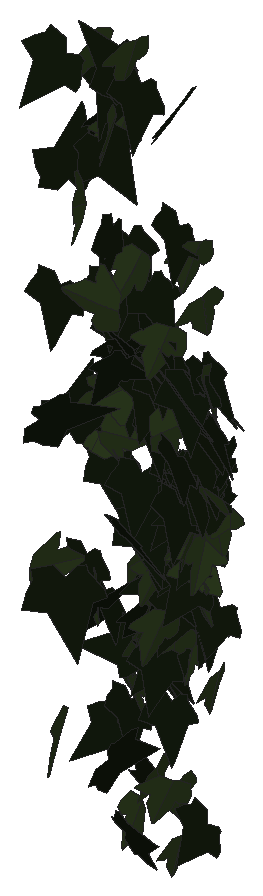
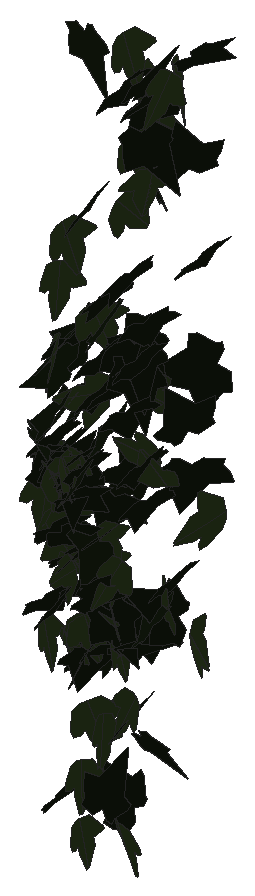
# SketchUp Ruby script. Lengths in inches.
U = 1.inch
M = Sketchup.active_model
def pt(a) = Geom::Point3d.new(a.map { |v| v * U })
def face(e, loops, mat)
  f = e.add_face(loops[0].map { |a| pt(a) })
  loops[1..].each { |l| e.add_face(l.map { |a| pt(a) }).erase! }
  f.material = f.back_material = mat if mat
  f
end
# faces: each face lists its corners as indices into pts; further lists are holes
def faces(e, pts, list, mat = nil) = list.each { |f| face(e, (f[0].is_a?(Array) ? f : [f]).map { |l| l.map { |i| pts[i] } }, mat) }
# xy, xz, yz: faces in a plane at the given z, y or x. An outline is a flat list of corners, or four numbers for a rectangle; further outlines are holes
def ring(l) = l.size == 4 ? [[l[0], l[1]], [l[2], l[1]], [l[2], l[3]], [l[0], l[3]]] : l.each_slice(2).to_a
def flat(e, list, mat, &to3) = list.each { |f| face(e, (f[0].is_a?(Array) ? f : [f]).map { |l| ring(l).map { |u, v| to3.(u, v) } }, mat) }
def xy(e, z, list, mat = nil) = flat(e, list, mat) { |x, y| [x, y, z] }
def xz(e, y, list, mat = nil) = flat(e, list, mat) { |x, z| [x, y, z] }
def yz(e, x, list, mat = nil) = flat(e, list, mat) { |y, z| [x, y, z] }
def lines(e, pts, list) = list.each { |a, b| e.add_line(pt(pts[a]), pt(pts[b])) }
# prism: a flat outline (further loops are holes) pulled along v
def prism(e, loops, v, mat = nil)
  f = face(e, loops, mat); d = Geom::Vector3d.new(v.map { |x| x * U })
  f.pushpull(f.normal.samedirection?(d) ? d.length : -d.length)
end
def box(e, o, s, mat = nil) = prism(e, [[o, [o[0] + s[0], o[1], o[2]], [o[0] + s[0], o[1] + s[1], o[2]], [o[0], o[1] + s[1], o[2]]]], [0, 0, s[2]], mat)
def at(x, y, z, deg = 0) = Geom::Transformation.translation(pt([x, y, z])) * Geom::Transformation.rotation(ORIGIN, Z_AXIS, deg.degrees)
def axes(o, x, y, z) = Geom::Transformation.new([*x, 0, *y, 0, *z, 0, *pt(o).to_a, 1])
def part(name) = M.definitions.add(name)
# library, detail: a bought-in or finely detailed component or shape, given as its bounding box
def library(name, o, s) = part(name).tap { |d| box(d.entities, o, s) }
def detail(e, o, s) = box(e.add_group.entities, o, s)
def put(e, d, t, mat = nil) = e.add_instance(d, t).tap { |i| i.material = mat if mat }
def group(e, t, mat = nil) = e.add_group.tap { |g| g.transformation = t; g.material = mat if mat }.entities
root = M.entities
M.materials.add("efeu1").color = [18, 25, 13]
M.materials.add("efeu2").color = [43, 57, 29]
c1 = part("ivyleaf_9")
p = [[1.54,2.16,1.25],[1.36,2.04,1.19],[-0.21,0.99,0.68],[-0.71,1.11,0.82],[-0.85,0.86,0.67],[-0.8,0.17,0.21],
  [-0.9,-0.01,0.1],[-0.67,-0.16,-0.02],[-0.08,-0.08,-0.05],[-0.03,-0.6,-0.4],[0.65,-0.88,-0.66],[0.83,-0.6,-0.49],
  [1.29,-0.42,-0.43],[1.8125,-0.07,-0.26],[1.21,0.44,0.15]]
faces(c1.entities,p,[[0,1,2,3,4,5,6,7,8,9,10,11,12,13,14]],"efeu1")
c2 = part("ivyleaf_10")
p = [[0,0.5,-0.03],[-0.0625,2.02,-0.43],[-0.19,2.01,-0.46],[-0.54,1.05,-0.29],[-0.52,0.625,-0.18],[-0.83,0.76,-0.28],
  [-1.16,0.64,-0.33],[-1.15,0.33,-0.24],[-0.77,-0.39,0.02],[-0.3,-0.51,0.16],[0.04,-0.48,0.23],[-0.02,2.01,-0.4375],
  [-0.06,2.01,-0.43],[0.04,-0.49,0.23],[0.67,-0.49,0.14],[1.38,0.36,-0.2],[1.375,0.51,-0.24],[0.81,0.65,-0.19],
  [0.62,0.59,-0.15],[0.6,1.09,-0.28],[0.5,1.23,-0.31]]
faces(c2.entities,p,[[0,1,2,3,4,5,6,7,8,9,10],[11,12,0,13,14,15,16,17,18,19,20]],"efeu2")
put(root,c1,axes([514.97,129.23,242.45],[-0.5414,-0.75563,0.39473],[-0.12929,-0.38942,-0.92279],[0.84266,-0.54524,0.11202]))
put(root,c1,axes([514.85,129.82,225.01],[-0.45465,-0.37518,0.81195],[0.67967,0.44717,0.5872],[-0.58144,0.81608,0.05152]))
put(root,c1,axes([514.61,131.17,218.48],[0.05064,-0.90044,0.13314],[0.04547,-0.13068,-0.90108],[0.9091,0.0567,0.03766]))
put(root,c2,axes([514.66,131.8,223.52],[0.87506,0.12632,-0.31002],[0.2718,0.23843,0.86434],[0.19543,-0.89722,0.18604]))
put(root,c2,axes([514.94,131.0625,241.9375],[-0.15471,-0.76586,-0.63412],[0.22492,0.59816,-0.7773],[0.96853,-0.26124,0.07922]))
put(root,c1,axes([515.54,131.78,210.88],[-0.86529,0.01971,0.04934],[-0.04909,0.01165,-0.86545],[-0.02034,-0.86662,-0.01051]))
put(root,c2,axes([514.6,131.39,217.29],[0.43583,-0.26126,0.83715],[0.76358,-0.34669,-0.50572],[0.43129,0.87782,0.04942]))
put(root,c1,axes([514.89,132.79,224.55],[0.10903,-0.92058,-0.06337],[0.00755,0.0647,-0.92689],[0.92273,0.10824,0.01507]))
put(root,c1,axes([515.29,129.18,237.07],[-0.6384,-0.40319,0.70228],[0.63185,0.3113,0.7531],[-0.50648,0.89657,0.05433]))
put(root,c2,axes([515.2,127.61,219.7],[0.0344,0.13379,1.09212],[-0.07348,1.09049,-0.13128],[-1.09782,-0.06879,0.043]))
put(root,c1,axes([514.98,132.31,222.63],[0.06062,-0.8883,-0.25008],[0.01661,0.25162,-0.88977],[0.92268,0.05383,0.03245]))
put(root,c1,axes([514.93,132,216.61],[0.21538,-0.81471,0.45489],[0.21685,-0.41037,-0.83764],[0.90755,0.2914,0.09219]))
put(root,c1,axes([515.85,131.41,239.32],[-0.28255,0.7891,-0.54165],[-0.00408,-0.56575,-0.82208],[-0.9571,-0.23055,0.16341]))
put(root,c2,axes([515.35,131.61,237.64],[0.32424,0.92853,0.11872],[0.01296,0.12118,-0.98313],[-0.936,0.32333,0.02751]))
put(root,c1,axes([515.3,132.05,230.875],[-0.17289,-0.9389,-0.10082],[0.02891,0.09719,-0.95463],[0.94386,-0.17496,0.01078]))
put(root,c1,axes([515.18,130.18,216.17],[0.12808,0.95405,-0.29052],[-0.0127,0.29444,0.96133],[0.99722,-0.11879,0.04955]))
put(root,c1,axes([515.38,128.4375,232.29],[-0.07402,-0.94076,0.22442],[0.05681,-0.22892,-0.94088],[0.96549,-0.05865,0.07256]))
put(root,c1,axes([515.48,132.44,229.15],[-0.02649,-0.94817,0.06026],[-0.02884,-0.05946,-0.94815],[0.94964,-0.02826,-0.02711]))
put(root,c2,axes([516.39,130.83,226.77],[0.47667,0.19364,-0.82272],[-0.7974,-0.21014,-0.51146],[-0.28023,0.92733,0.0559]))
put(root,c2,axes([515.93,132.66,206.69],[0.81961,-0.50896,-0.13471],[-0.1147,0.07064,-0.96478],[0.51384,0.8276,-0.00049]))
put(root,c2,axes([515.78,132.47,212.75],[-0.73675,0.41996,-0.20628],[0.19228,-0.07902,-0.84764],[-0.42654,-0.76099,-0.02582]))
put(root,c1,axes([515.47,127.3,226.75],[0.12289,0.59882,-0.92124],[0.10809,0.9159,0.60977],[1.09343,-0.15785,0.04326]))
put(root,c1,axes([515.76,132.68,226.73],[-0.16512,-0.92005,-0.12111],[0.01846,0.11973,-0.93474],[0.9278,-0.16612,-0.00295]))
put(root,c1,axes([516.35,131.24,241.11],[-0.23137,-0.96646,0.15669],[0.03489,0.15277,0.99377],[-0.97846,0.23398,-0.00162]))
put(root,c1,axes([516.3,131.25,227.98],[0.04211,0.93106,-0.20242],[-0.04863,-0.20026,-0.93122],[-0.95157,0.05144,0.03863]))
put(root,c2,axes([516.1875,131.52,238.78],[-0.39852,-0.83351,0.36406],[-0.00243,-0.3965,-0.91043],[0.90955,-0.36627,0.15709]))
put(root,c1,axes([516.67,131.9,214.6],[-0.56947,0.06456,0.67096],[-0.6084,-0.42736,-0.47525],[0.29018,-0.76931,0.32031]))
put(root,c2,axes([515.38,131.66,224.26],[0.06235,-0.00685,-0.9447],[0.91852,-0.22102,0.06222],[-0.22099,-0.9206,-0.00791]))
put(root,c1,axes([516.57,131.15,228.88],[0.2762,0.79679,-0.45461],[-0.21491,-0.40536,-0.84104],[-0.89183,0.34445,0.06188]))
put(root,c1,axes([515.99,132.21,233.02],[0.23414,-0.89814,-0.26951],[-0.00466,0.27666,-0.92603],[0.93769,0.22563,0.06269]))
put(root,c1,axes([516.03,132.18,211.84],[0.13673,-0.89736,0.27387],[0.03513,-0.27167,-0.9077],[0.93756,0.14104,-0.00593]))
put(root,c1,axes([516.18,131.26,240.69],[-0.18051,-0.88959,0.42906],[0.01216,-0.43814,-0.90329],[0.98758,-0.15721,0.08955]))
put(root,c2,axes([516.41,127.29,213.25],[0.4917,-0.77823,0.62119],[0.37306,-0.49837,-0.91964],[0.92323,0.61586,0.04077]))
put(root,c2,axes([516.58,132.31,218.76],[-0.19307,-0.61993,-0.68087],[0.27339,0.62571,-0.64723],[0.87929,-0.33067,0.05174]))
put(root,c2,axes([516.71,132.04,215.13],[0.17918,-0.85594,0.12987],[0.08527,-0.11453,-0.87248],[0.86153,0.18935,0.05934]))
put(root,c1,axes([516.82,132.91,207.76],[0.67382,-0.38153,0.53566],[-0.44923,0.29309,0.77384],[-0.48031,-0.80936,0.02771]))
put(root,c1,axes([517.03,132.11,216.52],[-0.10345,0.71078,-0.53068],[-0.02404,-0.53633,-0.71366],[-0.88671,-0.06838,0.08126]))
put(root,c1,axes([517.11,130.51,228.63],[-0.02065,0.64551,-0.73056],[-0.06379,-0.73006,-0.64326],[-0.9728,0.03417,0.05769]))
put(root,c1,axes([517.3125,133.54,217.75],[-0.45346,-0.42712,0.63768],[-0.47642,-0.42406,-0.62282],[0.60175,-0.65761,-0.01256]))
put(root,c1,axes([516.34,130.89,229.09],[0.86994,-0.31244,0.24362],[0.23084,-0.07799,-0.92434],[0.322,0.90004,0.00448]))
put(root,c2,axes([517.07,131.83,216.31],[0.46226,-0.76046,0.01149],[0.006,-0.0098,-0.88993],[0.76052,0.4623,0.00004]))
put(root,c2,axes([517.27,130.78,242.86],[-0.12238,-0.98728,0.13819],[-0.03293,-0.13515,-0.99471],[0.99636,-0.12573,-0.0159]))
put(root,c2,axes([517.64,132.98,216.11],[-0.57716,-0.60238,0.2892],[-0.08934,-0.30914,-0.82223],[0.6622,-0.56673,0.14112]))
put(root,c1,axes([517.24,131.34,223.05],[-0.16094,-0.9143,0.00882],[-0.00134,-0.00872,-0.92836],[0.91434,-0.16095,0.00019]))
put(root,c1,axes([517.19,128.9375,239.39],[0.15979,-0.74998,-0.71436],[-0.12003,0.70453,-0.76651],[1.02877,0.19869,0.02152]))
put(root,c1,axes([517.02,131.8125,214.74],[0.70082,-0.53811,0.023],[0.0249,-0.00533,-0.88351],[0.53802,0.70118,0.01093]))
put(root,c1,axes([517.26,131.27,240.92],[-0.02152,-0.98939,0.15928],[-0.0298,-0.15861,-0.98928],[1.00169,-0.02598,-0.02601]))
put(root,c1,axes([517.3125,132.02,226.89],[-0.14362,-0.88816,0.27106],[0.024,-0.27774,-0.89734],[0.92829,-0.13023,0.06514]))
put(root,c1,axes([517.24,132.63,227.23],[0.12082,-0.9372,-0.04866],[-0.00157,0.04886,-0.94495],[0.93846,0.12074,0.00469]))
put(root,c2,axes([517.68,128.84,240.34],[0.54098,-0.89201,-0.14499],[-0.07352,0.12498,-1.04324],[0.90072,0.54595,0.00193]))
put(root,c1,axes([517.26,131.9375,231.51],[0.23885,-0.888,-0.27966],[0.05806,0.30236,-0.9105],[0.92919,0.20937,0.12878]))
put(root,c1,axes([517.46,133,214.84],[-0.22149,-0.76154,-0.47931],[0.14821,0.456,-0.79299],[0.88753,-0.2662,0.01281]))
put(root,c1,axes([517.25,132.09,224.87],[0.23665,-0.79116,0.44836],[0.1751,-0.41498,-0.82468],[0.89236,0.29124,0.04291]))
put(root,c1,axes([517.96,132.43,214.96],[-0.66324,-0.5663,0.16308],[-0.1201,-0.11048,-0.8721],[0.57695,-0.674,0.00593]))
put(root,c1,axes([516.99,130.78,206.74],[0.78907,-0.0583,-0.62726],[0.62995,0.06764,0.78617],[-0.00338,-1.00574,0.08923]))
put(root,c1,axes([517.33,132.1,230.17],[0.44208,-0.84127,0.09918],[0.03185,-0.09528,-0.95022],[0.8465,0.44294,-0.01604]))
put(root,c1,axes([518.03,131.77,219.33],[0.19596,0.77834,0.42438],[-0.06605,0.44623,-0.78792],[-0.88405,0.13919,0.15293]))
put(root,c1,axes([517.59,126.1,220.625],[-0.39077,-0.89375,-0.59578],[0.24903,0.54133,-0.97539],[1.04486,-0.46327,0.00965]))
put(root,c1,axes([517.68,132.05,215.04],[0.50822,-0.64767,-0.5035],[-0.26839,0.42842,-0.82201],[0.77521,0.57293,0.0455]))
put(root,c1,axes([517.67,131.14,221.32],[-0.45073,-0.54286,-0.6934],[0.4979,0.4854,-0.70366],[0.72635,-0.66959,0.05207]))
put(root,c1,axes([517.7,132.23,228.45],[0.01263,-0.94916,0.04458],[0.00488,-0.04452,-0.94923],[0.95019,0.01284,0.00428]))
put(root,c2,axes([518.24,131.36,219.29],[-0.23803,-0.78157,0.42887],[-0.03388,-0.43564,-0.81272],[0.89086,-0.22539,0.08368]))
put(root,c2,axes([518.22,132.58,206.02],[-0.0103,-0.84798,0.00435],[-0.00068,-0.00435,-0.84804],[0.84799,-0.0103,-0.00063]))
put(root,c2,axes([518.33,132.24,215.59],[-0.54684,-0.69843,0.08079],[-0.05725,-0.05777,-0.88699],[0.70075,-0.54975,-0.00943]))
put(root,c1,axes([517.98,128.55,235.76],[-0.66293,0.00185,-0.81514],[0.80974,-0.1192,-0.65882],[-0.09364,-1.0439,0.07378]))
put(root,c1,axes([518.28,133.125,221.99],[-0.57042,-0.69898,0.19822],[-0.07979,-0.19023,-0.90039],[0.72215,-0.57314,0.0571]))
put(root,c2,axes([518.3125,132.47,208.69],[-0.169,-0.85058,-0.14809],[0.02316,0.14637,-0.86719],[0.86306,-0.17048,-0.00573]))
put(root,c1,axes([518,132.89,223.4],[0.02001,-0.92729,-0.04151],[-0.01886,0.04111,-0.92733],[0.92803,0.02083,-0.01795]))
put(root,c1,axes([517.83,133.04,223.25],[0.506,-0.7704,0.08751],[0.02789,-0.08634,-0.9214],[0.77485,0.5062,-0.02398]))
put(root,c2,axes([518.51,131.36,229.84],[-0.52587,-0.69764,0.39663],[-0.06221,-0.43734,-0.85172],[0.80009,-0.49254,0.19447]))
put(root,c1,axes([517.84,129.1,221.93],[1.00558,-0.22039,-0.07497],[-0.07288,0.01767,-1.02945],[0.22109,1.00822,0.00166]))
put(root,c2,axes([518.81,125.52,238.61],[0.35696,-0.56862,-0.94553],[-0.50849,0.79717,-0.67137],[0.97918,0.62126,-0.00395]))
put(root,c2,axes([518.46,130.84,210.05],[0.08761,-0.8972,-0.33867],[0.03946,0.34317,-0.8989],[0.95818,0.0679,0.06798]))
put(root,c1,axes([518.66,132.47,223.11],[0.41723,0.74755,-0.33083],[-0.18742,-0.27406,-0.85564],[-0.79571,0.45653,0.02806]))
put(root,c2,axes([518.52,129.39,234.09],[-0.27097,-0.67442,0.73419],[0.18396,-0.78158,-0.65007],[0.97981,-0.03977,0.32509]))
put(root,c2,axes([518.57,132.23,222.57],[0.20815,-0.84209,-0.33055],[0.07654,0.35436,-0.85456],[0.9014,0.16437,0.14889]))
put(root,c1,axes([518.13,131.71,219.42],[0.50315,-0.64277,-0.39943],[-0.00815,0.47503,-0.77469],[0.75673,0.43249,0.25724]))
put(root,c2,axes([518.48,132.99,214.97],[0.81816,-0.32092,0.07829],[0.07032,-0.03514,-0.87882],[0.32276,0.82114,-0.00701]))
put(root,c2,axes([518.75,133.01,223.23],[0.29693,-0.87488,0.04478],[0.00788,-0.04461,-0.92387],[0.87599,0.29695,-0.00686]))
put(root,c1,axes([518.69,132.31,217.29],[-0.37658,-0.77201,0.22239],[-0.02307,-0.23511,-0.85525],[0.80307,-0.36877,0.07971]))
put(root,c2,axes([519.07,133.24,222.84],[-0.23675,-0.52738,0.70551],[-0.20491,-0.67753,-0.57523],[0.85667,-0.30781,0.05739]))
put(root,c1,axes([519.07,132.74,219.88],[-0.66467,-0.58662,0.14228],[-0.11182,-0.08831,-0.88648],[0.59318,-0.67397,-0.00769]))
put(root,c2,axes([519.03,130.46,217.37],[-0.27274,-0.85919,0.40955],[-0.01763,-0.4214,-0.89578],[0.95164,-0.25405,0.10078]))
put(root,c1,axes([518.76,130.73,215.57],[-0.17744,-0.86624,0.11328],[-0.00132,-0.11533,-0.88396],[0.87361,-0.17612,0.02167]))
put(root,c2,axes([518.99,132.19,223.36],[0.81722,-0.39496,-0.12894],[-0.10881,0.07113,-0.90751],[0.40098,0.82427,0.01653]))
put(root,c2,axes([519.19,132.33,222.95],[-0.51019,-0.75326,0.02026],[-0.01275,-0.01584,-0.90978],[0.75343,-0.51035,-0.00167]))
put(root,c1,axes([518.96,132.66,223.01],[-0.31869,-0.73457,0.46803],[-0.03774,-0.48626,-0.78888],[0.87019,-0.29011,0.13719]))
put(root,c2,axes([518.7,130.86,225.79],[0.03852,0.1013,-1.03408],[0.61138,0.83449,0.10452],[0.84012,-0.61192,-0.02865]))
put(root,c1,axes([519.35,131.86,222.52],[-0.89304,-0.19626,-0.10725],[0.10711,0.01224,-0.91428],[0.19633,-0.89937,0.01096]))
put(root,c1,axes([518.85,131.76,234.76],[0.0888,-0.88752,0.40494],[0.01449,-0.40537,-0.89164],[0.97543,0.08682,-0.02362]))
put(root,c2,axes([519.3,131.95,220.63],[0.4365,-0.7904,-0.01328],[-0.01478,0.00701,-0.90287],[0.79038,0.43665,-0.00955]))
put(root,c1,axes([519.3,133.17,220.21],[-0.4751,-0.7387,0.22055],[-0.07917,-0.21095,-0.87708],[0.76684,-0.47945,0.04609]))
put(root,c2,axes([518.89,132.64,218.05],[-0.52969,0.37295,-0.64477],[0.52338,-0.3766,-0.6478],[-0.52999,-0.74463,0.00469]))
put(root,c2,axes([519.42,132.14,233.76],[-0.23124,-0.9054,0.24803],[-0.00585,-0.25404,-0.93283],[0.93874,-0.22461,0.05528]))
put(root,c2,axes([519.48,132.48,220.72],[0.19753,0.30725,-0.87481],[-0.40502,-0.776,-0.364],[-0.83406,0.44959,-0.03042]))
put(root,c2,axes([519.42,132.1875,218.99],[0.68646,0.48259,-0.38033],[-0.33552,-0.18332,-0.8382],[-0.51475,0.76306,0.03916]))
put(root,c1,axes([519.11,130.96,213.375],[-0.09438,-0.86531,-0.13613],[0.00908,0.13594,-0.87043],[0.87591,-0.09465,-0.00564]))
put(root,c1,axes([519.3125,132.27,218.54],[-0.43603,-0.69154,0.35139],[-0.02324,-0.39127,-0.79887],[0.77535,-0.40062,0.17366]))
put(root,c2,axes([519.64,130.21,210.06],[-0.553,-0.67674,0.33486],[-0.22083,-0.25195,-0.87388],[0.72204,-0.59536,-0.01081]))
put(root,c1,axes([519.13,133.28,216.6],[0.12847,-0.86186,0.21474],[0.02605,-0.21322,-0.87136],[0.88783,0.13097,-0.0055]))
put(root,c1,axes([519.05,132.68,225.79],[0.51554,-0.76888,-0.16119],[-0.0573,0.15548,-0.92492],[0.7835,0.51729,0.03842]))
put(root,c1,axes([519.58,126.49,212.95],[-0.16488,0.31858,-1.017],[-0.41351,0.92935,0.35816],[0.98223,0.44472,-0.01993]))
put(root,c1,axes([519.45,132.73,207.17],[-0.25711,-0.68546,0.53173],[-0.06697,-0.53725,-0.72497],[0.86493,-0.24536,0.10192]))
put(root,c1,axes([519.86,132.48,221.95],[0.20864,0.14702,0.91682],[-0.83585,-0.37949,0.25107],[0.40437,-0.86027,0.04593]))
put(root,c2,axes([519.11,133.3,222.25],[-0.10423,-0.07776,-0.90568],[0.65695,-0.63651,-0.02095],[-0.62827,-0.65267,0.12834]))
put(root,c2,axes([519.44,132,222.85],[-0.77019,-0.17374,-0.47536],[0.4849,-0.00534,-0.7837],[0.14499,-0.90505,0.09587]))
put(root,c1,axes([519.61,133.37,216.82],[-0.32245,-0.82781,0.14276],[0.0219,-0.16115,-0.88497],[0.83974,-0.31366,0.0779]))
put(root,c2,axes([519.9,131.97,231.61],[-0.2473,-0.89571,-0.26018],[0.05083,0.25583,-0.92904],[0.93135,-0.2518,-0.01839]))
put(root,c1,axes([519.52,130.9375,222.63],[0.04366,-0.8872,0.30401],[0.00177,-0.30426,-0.88818],[0.93784,0.04187,-0.01248]))
put(root,c1,axes([519.21,132.46,227.55],[0.75312,-0.52571,0.14139],[0.19452,0.03445,-0.90803],[0.50845,0.7655,0.13796]))
put(root,c1,axes([519.57,132.22,223.54],[0.08726,-0.9231,0.08257],[0.01791,-0.08124,-0.92716],[0.92661,0.0885,0.01014]))
put(root,c1,axes([520.52,132.06,222.8],[-0.84695,-0.15141,0.42886],[-0.40937,-0.1411,-0.85829],[0.19813,-0.93879,0.05984]))
put(root,c1,axes([519.39,132.97,225.52],[0.47659,-0.755,0.24779],[0.15302,-0.19633,-0.89252],[0.77975,0.49999,0.0237]))
put(root,c1,axes([519.67,132.75,224.29],[0.0493,-0.91653,-0.07833],[0.02584,0.07979,-0.91736],[0.91951,0.0469,0.02998]))
put(root,c2,axes([519.96,132.03,220.37],[0.18016,0.82699,-0.40912],[-0.11598,-0.39324,-0.84596],[-0.91533,0.2126,0.02667]))
put(root,c1,axes([519.58,132.46,228.35],[0.53002,-0.76026,-0.21882],[-0.05279,0.22881,-0.92285],[0.78936,0.52578,0.08521]))
put(root,c1,axes([520.52,129.5,241.64],[-0.46516,0.90858,0.01759],[-0.00797,0.01568,-1.02073],[-0.90871,-0.46522,-0.00005]))
put(root,c2,axes([520.25,131.83,227.98],[-0.5579,0.6618,0.41279],[-0.27819,0.30531,-0.86546],[-0.72868,-0.62325,0.01436]))
put(root,c2,axes([520.8,131.85,222.39],[0.08526,0.10533,-0.92906],[-0.90467,0.24501,-0.05524],[0.23625,0.90021,0.12374]))
put(root,c1,axes([520.45,132.91,224.16],[-0.80239,0.33823,-0.27243],[0.20962,-0.19964,-0.86525],[-0.38036,-0.82353,0.09786]))
put(root,c1,axes([519.9,131.23,228.14],[-0.1469,-0.96307,-0.15309],[0.02377,0.15124,-0.97421],[0.97487,-0.14881,0.00068]))
put(root,c1,axes([519.65,130.67,224.98],[0.18372,-0.73858,0.56581],[0.21748,-0.52666,-0.7581],[0.90462,0.27661,0.06735]))
put(root,c2,axes([520.23,132.45,221.57],[-0.61098,-0.66415,-0.12514],[0.13488,0.04547,-0.89989],[0.66224,-0.62201,0.06783]))
put(root,c2,axes([521.12,124.45,235.16],[0.01356,0.05992,1.19884],[-1.18498,-0.19054,0.02293],[0.19143,-1.18368,0.05699]))
put(root,c1,axes([519.52,130.77,227.81],[0.55005,-0.5863,0.62123],[0.41985,-0.45791,-0.80391],[0.74391,0.69195,-0.00563]))
put(root,c2,axes([520.52,132.06,214.55],[0.16861,-0.88368,-0.08123],[-0.01647,0.07955,-0.89962],[0.88725,0.16941,-0.00126]))
